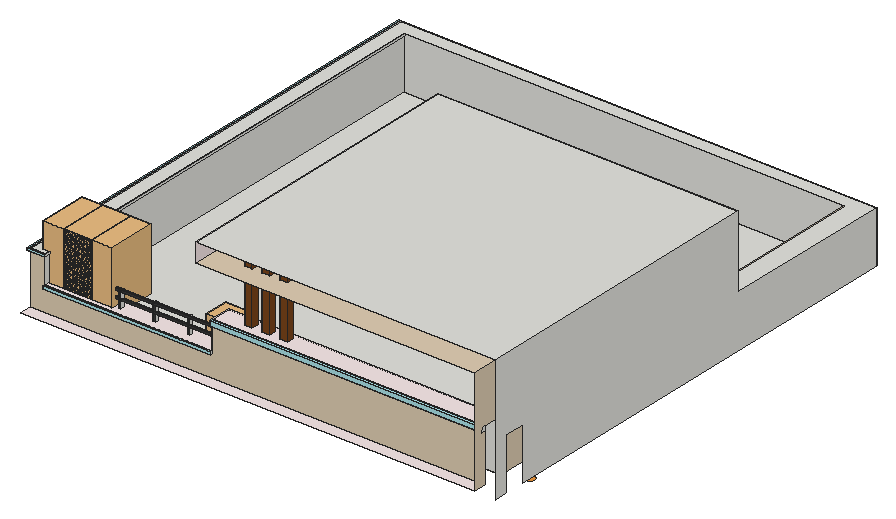
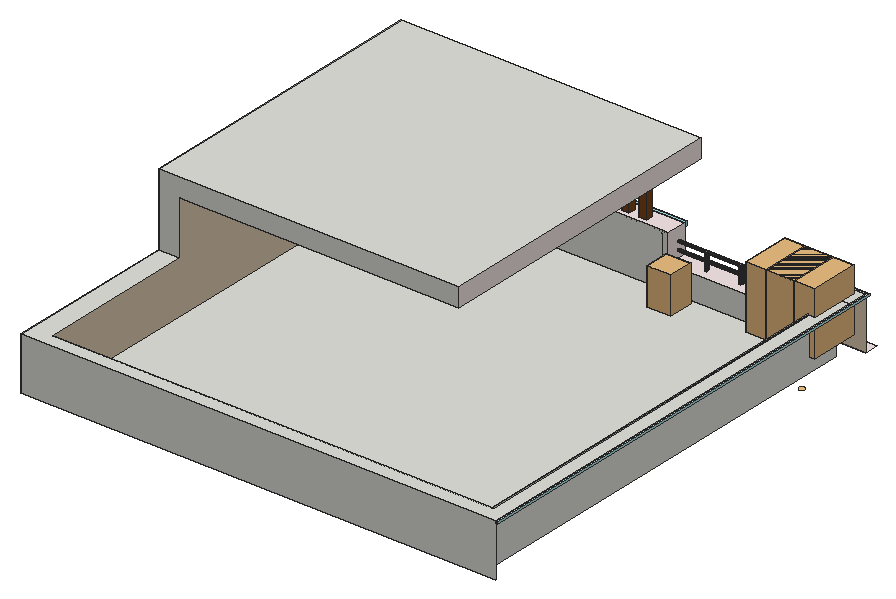
# SketchUp Ruby script. Lengths in inches.
U = 1.inch
M = Sketchup.active_model
def pt(a) = Geom::Point3d.new(a.map { |v| v * U })
def face(e, loops, mat)
  f = e.add_face(loops[0].map { |a| pt(a) })
  loops[1..].each { |l| e.add_face(l.map { |a| pt(a) }).erase! }
  f.material = f.back_material = mat if mat
  f
end
# faces: each face lists its corners as indices into pts; further lists are holes
def faces(e, pts, list, mat = nil) = list.each { |f| face(e, (f[0].is_a?(Array) ? f : [f]).map { |l| l.map { |i| pts[i] } }, mat) }
# xy, xz, yz: faces in a plane at the given z, y or x. An outline is a flat list of corners, or four numbers for a rectangle; further outlines are holes
def ring(l) = l.size == 4 ? [[l[0], l[1]], [l[2], l[1]], [l[2], l[3]], [l[0], l[3]]] : l.each_slice(2).to_a
def flat(e, list, mat, &to3) = list.each { |f| face(e, (f[0].is_a?(Array) ? f : [f]).map { |l| ring(l).map { |u, v| to3.(u, v) } }, mat) }
def xy(e, z, list, mat = nil) = flat(e, list, mat) { |x, y| [x, y, z] }
def xz(e, y, list, mat = nil) = flat(e, list, mat) { |x, z| [x, y, z] }
def yz(e, x, list, mat = nil) = flat(e, list, mat) { |y, z| [x, y, z] }
def lines(e, pts, list) = list.each { |a, b| e.add_line(pt(pts[a]), pt(pts[b])) }
# prism: a flat outline (further loops are holes) pulled along v
def prism(e, loops, v, mat = nil)
  f = face(e, loops, mat); d = Geom::Vector3d.new(v.map { |x| x * U })
  f.pushpull(f.normal.samedirection?(d) ? d.length : -d.length)
end
def box(e, o, s, mat = nil) = prism(e, [[o, [o[0] + s[0], o[1], o[2]], [o[0] + s[0], o[1] + s[1], o[2]], [o[0], o[1] + s[1], o[2]]]], [0, 0, s[2]], mat)
def at(x, y, z, deg = 0) = Geom::Transformation.translation(pt([x, y, z])) * Geom::Transformation.rotation(ORIGIN, Z_AXIS, deg.degrees)
def axes(o, x, y, z) = Geom::Transformation.new([*x, 0, *y, 0, *z, 0, *pt(o).to_a, 1])
def part(name) = M.definitions.add(name)
# library, detail: a bought-in or finely detailed component or shape, given as its bounding box
def library(name, o, s) = part(name).tap { |d| box(d.entities, o, s) }
def detail(e, o, s) = box(e.add_group.entities, o, s)
def put(e, d, t, mat = nil) = e.add_instance(d, t).tap { |i| i.material = mat if mat }
def group(e, t, mat = nil) = e.add_group.tap { |g| g.transformation = t; g.material = mat if mat }.entities
root = M.entities
M.materials.add("Generic\#1").color = [121, 68, 27]
M.materials.add("Generic\#2").color = [245, 199, 133]
M.materials.add("Generic\#4").color = [232, 149, 60]
M.materials.add("Generic\#6").color = [223, 205, 179]
M.materials.add("Generic\#7").color = [171, 227, 232]
M.materials.add("Generic\#9").color = [246, 231, 231]
M.materials.add("[Color M07]").color = [58, 58, 58]
c1 = library("Raised potted plant",[1.65,0,0],[13.63,13.63,20.73])
c2 = library("Plant+2 (1)",[-9.13,-9.52,0],[51.76,51.77,66.88])
c3 = library("Tlon Light 450 Ceiling 152 006",[-8.86,-8.86,-3.78],[17.72,17.72,3.56])
xy(root,545.1875,[[26.07,107.35,25.33,107.49,24.65,107.8,24.07,108.29,23.64,108.9,23.39,109.61,23.32,110.36,23.46,111.1,23.77,111.78,24.26,112.35,24.875,112.78,25.58,113.03,26.33,113.1,27.07,112.97,27.75,112.65,28.32,112.16,28.75,111.55,29,110.84,29.07,110.1,28.9375,109.36,28.62,108.68,28.13,108.1,27.52,107.67,26.8125,107.42],[102.38,107.35,101.64,107.49,100.96,107.8,100.39,108.29,99.96,108.9,99.7,109.61,99.64,110.36,99.77,111.1,100.09,111.78,100.57,112.35,101.1875,112.78,101.89,113.03,102.64,113.1,103.38,112.97,104.06,112.65,104.63,112.16,105.0625,111.55,105.32,110.84,105.38,110.1,105.25,109.36,104.93,108.68,104.45,108.1,103.83,107.67,103.125,107.42],[179.07,107.35,178.33,107.49,177.65,107.8,177.07,108.29,176.64,108.9,176.39,109.61,176.32,110.36,176.46,111.1,176.77,111.78,177.26,112.35,177.875,112.78,178.58,113.03,179.33,113.1,180.07,112.97,180.75,112.65,181.32,112.16,181.75,111.55,182,110.84,182.07,110.1,181.9375,109.36,181.62,108.68,181.13,108.1,180.52,107.67,179.8125,107.42]],"Generic\#2")
xy(root,545.1875,[[327.25,107.79,326.17,108.08,325.19,108.65,324.4,109.45,323.83,110.42,323.54,111.51,323.55,112.64,323.84,113.72,324.4,114.7,325.2,115.49,326.18,116.05,327.26,116.34,328.39,116.34,329.48,116.05,330.45,115.48,331.25,114.6875,331.81,113.71,332.1,112.625,332.1,111.5,331.8,110.41,331.24,109.4375,330.44,108.64,329.47,108.08,328.38,107.79],[417.81,107.79,416.73,108.08,415.75,108.65,414.96,109.45,414.4,110.42,414.11,111.51,414.11,112.64,414.4,113.72,414.97,114.7,415.76,115.49,416.74,116.05,417.83,116.34,418.95,116.34,420.04,116.05,421.01,115.48,421.81,114.6875,422.37,113.71,422.66,112.625,422.66,111.5,422.37,110.41,421.8,109.4375,421,108.64,420.03,108.08,418.94,107.79],[487.25,107.79,486.17,108.08,485.19,108.65,484.4,109.45,483.83,110.42,483.54,111.51,483.55,112.64,483.84,113.72,484.4,114.7,485.2,115.49,486.18,116.05,487.26,116.34,488.39,116.34,489.48,116.05,490.45,115.48,491.25,114.6875,491.81,113.71,492.1,112.625,492.1,111.5,491.8,110.41,491.24,109.4375,490.44,108.64,489.47,108.08,488.38,107.79]],"Generic\#4")
xy(root,563.5,[[17.125,76.4375,485.375,531.65]])
xy(root,563.5,[[2.3125,41,485.375,54.5625]],"Generic\#9")
xy(root,586.375,[[17.125,52.375,195.51,54.5625]])
xy(root,589.5625,[[53.47,63.23,55.65,65.98],[89.68,63.23,91.87,65.98],[125.9,63.23,128.08,65.98],[162.11,63.23,164.3,65.98]])
xy(root,589.5625,[[17.125,52.375,195.51,54.5625]],"Generic\#7")
xy(root,589.5625,[[[17.125,54.5625,195.51,76.4375],[162.11,63.23,164.3,65.98],[125.9,63.23,128.08,65.98],[89.68,63.23,91.87,65.98],[53.47,63.23,55.65,65.98]]],"Generic\#9")
xy(root,607.28,[[53.47,63.23,55.65,65.98],[89.68,63.23,91.87,65.98],[125.9,63.23,128.08,65.98],[162.11,63.23,164.3,65.98]],"[Color M07]")
xy(root,615,[[195.51,50.875,485.375,54.5625]])
xy(root,617.375,[[0,52.5,2.3125,546.8125],[2.3125,52.5,2.3125,54.5625,17.125,54.5625,17.125,531.65,18.6875,531.65,18.6875,52.5]])
xy(root,619.375,[[0,52.5,18.6875,52.5,18.6875,531.65,17.125,531.65,17.125,54.5625,2.3125,54.5625,2.3125,546.8125,0,546.8125],[2.3125,54.5625,17.125,76.4375],[2.3125,76.4375,17.125,76.4375,17.125,531.65,485.375,531.65,485.375,363.375,507.875,363.375,507.875,546.8125,2.3125,546.8125]])
xy(root,619.375,[[195.51,50.875,485.375,54.5625]],"Generic\#7")
xy(root,619.375,[[[195.51,54.5625,485.375,76.4375],[222.76,63.63,230.88,70.88],[241.38,63.63,249.51,70.88],[260.01,63.63,268.13,70.88]]],"Generic\#9")
xy(root,676.25,[[205.79,89.28,204.45,89.45,203.2,89.97,202.125,90.79,201.3,91.87,200.78,93.12,200.6,94.46,200.78,95.81,201.3,97.06,202.125,98.13,203.2,98.96,204.45,99.47,205.79,99.65,207.13,99.47,208.39,98.96,209.46,98.13,210.28,97.06,210.8,95.81,210.98,94.46,210.8,93.12,210.28,91.87,209.46,90.79,208.39,89.97,207.13,89.45]])
xy(root,676.25,[[[188.57,41,485.375,363.375],[291.79,89.28,293.13,89.45,294.39,89.97,295.46,90.79,296.28,91.87,296.8,93.12,296.98,94.46,296.8,95.81,296.28,97.06,295.46,98.13,294.39,98.96,293.13,99.47,291.79,99.65,290.45,99.47,289.2,98.96,288.125,98.13,287.3,97.06,286.78,95.81,286.6,94.46,286.78,93.12,287.3,91.87,288.125,90.79,289.2,89.97,290.45,89.45],[346.04,89.28,347.38,89.45,348.64,89.97,349.71,90.79,350.53,91.87,351.05,93.12,351.23,94.46,351.05,95.81,350.53,97.06,349.71,98.13,348.64,98.96,347.38,99.47,346.04,99.65,344.7,99.47,343.45,98.96,342.375,98.13,341.55,97.06,341.03,95.81,340.85,94.46,341.03,93.12,341.55,91.87,342.375,90.79,343.45,89.97,344.7,89.45],[400.29,89.28,401.63,89.45,402.89,89.97,403.96,90.79,404.78,91.87,405.3,93.12,405.48,94.46,405.3,95.81,404.78,97.06,403.96,98.13,402.89,98.96,401.63,99.47,400.29,99.65,398.95,99.47,397.7,98.96,396.625,98.13,395.8,97.06,395.28,95.81,395.1,94.46,395.28,93.12,395.8,91.87,396.625,90.79,397.7,89.97,398.95,89.45],[454.54,89.28,455.88,89.45,457.14,89.97,458.21,90.79,459.03,91.87,459.55,93.12,459.73,94.46,459.55,95.81,459.03,97.06,458.21,98.13,457.14,98.96,455.88,99.47,454.54,99.65,453.2,99.47,451.95,98.96,450.875,98.13,450.05,97.06,449.53,95.81,449.35,94.46,449.53,93.12,450.05,91.87,450.875,90.79,451.95,89.97,453.2,89.45],[205.79,89.28,207.13,89.45,208.39,89.97,209.46,90.79,210.28,91.87,210.8,93.12,210.98,94.46,210.8,95.81,210.28,97.06,209.46,98.13,208.39,98.96,207.13,99.47,205.79,99.65,204.45,99.47,203.2,98.96,202.125,98.13,201.3,97.06,200.78,95.81,200.6,94.46,200.78,93.12,201.3,91.87,202.125,90.79,203.2,89.97,204.45,89.45]]],"Generic\#6")
xy(root,678.8125,[[291.79,89.28,290.45,89.45,289.2,89.97,288.125,90.79,287.3,91.87,286.78,93.12,286.6,94.46,286.78,95.81,287.3,97.06,288.125,98.13,289.2,98.96,290.45,99.47,291.79,99.65,293.13,99.47,294.39,98.96,295.46,98.13,296.28,97.06,296.8,95.81,296.98,94.46,296.8,93.12,296.28,91.87,295.46,90.79,294.39,89.97,293.13,89.45],[346.04,89.28,344.7,89.45,343.45,89.97,342.375,90.79,341.55,91.87,341.03,93.12,340.85,94.46,341.03,95.81,341.55,97.06,342.375,98.13,343.45,98.96,344.7,99.47,346.04,99.65,347.38,99.47,348.64,98.96,349.71,98.13,350.53,97.06,351.05,95.81,351.23,94.46,351.05,93.12,350.53,91.87,349.71,90.79,348.64,89.97,347.38,89.45],[400.29,89.28,398.95,89.45,397.7,89.97,396.625,90.79,395.8,91.87,395.28,93.12,395.1,94.46,395.28,95.81,395.8,97.06,396.625,98.13,397.7,98.96,398.95,99.47,400.29,99.65,401.63,99.47,402.89,98.96,403.96,98.13,404.78,97.06,405.3,95.81,405.48,94.46,405.3,93.12,404.78,91.87,403.96,90.79,402.89,89.97,401.63,89.45],[454.54,89.28,453.2,89.45,451.95,89.97,450.875,90.79,450.05,91.87,449.53,93.12,449.35,94.46,449.53,95.81,450.05,97.06,450.875,98.13,451.95,98.96,453.2,99.47,454.54,99.65,455.88,99.47,457.14,98.96,458.21,98.13,459.03,97.06,459.55,95.81,459.73,94.46,459.55,93.12,459.03,91.87,458.21,90.79,457.14,89.97,455.88,89.45]],"Generic\#2")
xy(root,682.5,[[222.76,63.63,230.88,70.88],[241.38,63.63,249.51,70.88],[260.01,63.63,268.13,70.88]])
xy(root,696.375,[[188.57,41,507.875,363.375]])
xz(root,50.875,[[195.51,615,485.375,619.375]],"Generic\#7")
xz(root,52.375,[[17.125,586.375,195.51,589.5625]],"Generic\#7")
xz(root,52.5,[[0,617.375,18.6875,619.375]],"Generic\#7")
xz(root,54.5625,[[17.125,586.375,195.51,589.5625],[195.51,615,485.375,619.375],[2.3125,617.375,17.125,619.375]])
xz(root,54.5625,[[2.3125,563.5,485.375,563.5,485.375,615,195.51,615,195.51,586.375,17.125,586.375,17.125,617.375,2.3125,617.375]],"Generic\#6")
xz(root,63.23,[[53.47,589.5625,55.65,607.28],[89.68,589.5625,91.87,607.28],[125.9,589.5625,128.08,607.28],[162.11,589.5625,164.3,607.28]],"[Color M07]")
xz(root,63.63,[[222.76,619.375,230.88,682.5],[241.38,619.375,249.51,682.5],[260.01,619.375,268.13,682.5]],"Generic\#1")
xz(root,65.98,[[53.47,589.5625,55.65,607.28],[89.68,589.5625,91.87,607.28],[125.9,589.5625,128.08,607.28],[162.11,589.5625,164.3,607.28]],"[Color M07]")
xz(root,70.88,[[222.76,619.375,230.88,682.5],[241.38,619.375,249.51,682.5],[260.01,619.375,268.13,682.5]],"Generic\#1")
xz(root,76.4375,[[17.125,563.5,17.125,589.5625,195.51,589.5625,195.51,619.375,201.87,619.375,201.87,563.5],[201.87,563.5,485.375,619.375]])
xz(root,363.375,[[485.375,619.375,485.375,676.25,188.57,676.25,188.57,696.375,507.875,696.375,507.875,619.375]])
xz(root,531.65,[[17.125,563.5,485.375,563.5,485.375,619.375,18.6875,619.375,18.6875,617.375,17.125,617.375]])
xz(root,546.8125,[[2.3125,563.5,507.875,619.375],[0,617.375,2.3125,619.375]])
yz(root,0,[[52.5,617.375,546.8125,619.375]],"Generic\#7")
yz(root,2.3125,[[54.5625,617.375,546.8125,619.375]])
yz(root,17.125,[[76.4375,563.5,531.65,617.375],[[54.5625,589.5625,76.4375,617.375],[62.84,597.4,62.86,599.33,64.97,599.34,64.96,597.42],[62.84,605.34,62.86,607.27,64.97,607.28,64.96,605.36]],[54.5625,617.375,76.4375,619.375],[76.4375,617.375,531.65,619.375]])
yz(root,17.125,[[52.375,586.375,54.5625,589.5625]],"Generic\#7")
yz(root,18.6875,[[52.5,617.375,531.65,619.375]])
yz(root,53.47,[[63.23,589.5625,65.98,607.28]],"[Color M07]")
yz(root,55.65,[[63.23,589.5625,65.98,607.28]])
yz(root,89.68,[[63.23,589.5625,65.98,607.28]],"[Color M07]")
yz(root,91.87,[[63.23,589.5625,65.98,607.28]])
yz(root,125.9,[[63.23,589.5625,65.98,607.28]],"[Color M07]")
yz(root,128.08,[[63.23,589.5625,65.98,607.28]])
yz(root,162.11,[[63.23,589.5625,65.98,607.28]],"[Color M07]")
yz(root,164.3,[[63.23,589.5625,65.98,607.28]])
yz(root,188.57,[[41,676.25,363.375,696.375]],"Generic\#9")
yz(root,195.51,[[52.375,586.375,54.5625,589.5625],[62.84,597.4,64.96,597.42,64.97,599.34,62.86,599.33],[62.84,605.34,64.96,605.36,64.97,607.28,62.86,607.27]])
yz(root,195.51,[[50.875,615,54.5625,619.375]],"Generic\#7")
yz(root,195.51,[[[54.5625,589.5625,76.4375,619.375],[62.84,605.34,64.96,605.36,64.97,607.28,62.86,607.27],[62.84,597.4,64.96,597.42,64.97,599.34,62.86,599.33]]],"Generic\#9")
yz(root,222.76,[[63.63,619.375,70.88,682.5]],"Generic\#1")
yz(root,230.88,[[63.63,619.375,70.88,682.5]],"Generic\#1")
yz(root,241.38,[[63.63,619.375,70.88,682.5]],"Generic\#1")
yz(root,249.51,[[63.63,619.375,70.88,682.5]],"Generic\#1")
yz(root,260.01,[[63.63,619.375,70.88,682.5]],"Generic\#1")
yz(root,268.13,[[63.63,619.375,70.88,682.5]],"Generic\#1")
yz(root,485.375,[[50.875,615,54.5625,619.375]])
yz(root,485.375,[[41,563.5,41,676.25,363.375,676.25,363.375,619.375,531.65,619.375,531.65,563.5,76.4375,563.5,76.4375,619.375,50.875,619.375,50.875,615,54.5625,615,54.5625,563.5]],"Generic\#6")
yz(root,507.875,[[41,563.5,54.5625,563.5,54.5625,619.375,76.4375,619.375,76.4375,563.5,546.8125,563.5,546.8125,619.375,363.375,619.375,363.375,696.375,41,696.375]])
p = [[195.51,62.84,597.4],[195.51,62.86,599.33],[17.125,62.86,599.33],[17.125,62.84,597.4],[195.51,64.96,597.42],[17.125,64.96,597.42],
  [195.51,64.97,599.34],[17.125,64.97,599.34],[195.51,62.84,605.34],[195.51,62.86,607.27],[17.125,62.86,607.27],[17.125,62.84,605.34],
  [195.51,64.96,605.36],[17.125,64.96,605.36],[195.51,64.97,607.28],[17.125,64.97,607.28],[53.47,64.97,607.28],[55.65,64.97,607.28],
  [89.68,64.97,607.28],[91.87,64.97,607.28],[125.9,64.97,607.28],[128.08,64.97,607.28],[162.11,64.97,607.28],[164.3,64.97,607.28],
  [291.79,89.28,676.25],[290.45,89.45,676.25],[290.45,89.45,678.8125],[291.79,89.28,678.8125],[293.13,89.45,676.25],[293.13,89.45,678.8125],
  [346.04,89.28,676.25],[344.7,89.45,676.25],[344.7,89.45,678.8125],[346.04,89.28,678.8125],[347.38,89.45,676.25],[347.38,89.45,678.8125],
  [400.29,89.28,676.25],[398.95,89.45,676.25],[398.95,89.45,678.8125],[400.29,89.28,678.8125],[401.63,89.45,676.25],[401.63,89.45,678.8125],
  [454.54,89.28,676.25],[453.2,89.45,676.25],[453.2,89.45,678.8125],[454.54,89.28,678.8125],[455.88,89.45,676.25],[455.88,89.45,678.8125],
  [289.2,89.97,676.25],[289.2,89.97,678.8125],[294.39,89.97,676.25],[294.39,89.97,678.8125],[343.45,89.97,676.25],[343.45,89.97,678.8125],
  [348.64,89.97,676.25],[348.64,89.97,678.8125],[397.7,89.97,676.25],[397.7,89.97,678.8125],[402.89,89.97,676.25],[402.89,89.97,678.8125],
  [451.95,89.97,676.25],[451.95,89.97,678.8125],[457.14,89.97,676.25],[457.14,89.97,678.8125],[288.125,90.79,676.25],[288.125,90.79,678.8125],
  [295.46,90.79,676.25],[295.46,90.79,678.8125],[342.375,90.79,676.25],[342.375,90.79,678.8125],[349.71,90.79,676.25],[349.71,90.79,678.8125],
  [396.625,90.79,676.25],[396.625,90.79,678.8125],[403.96,90.79,676.25],[403.96,90.79,678.8125],[450.875,90.79,676.25],[450.875,90.79,678.8125],
  [458.21,90.79,676.25],[458.21,90.79,678.8125],[287.3,91.87,676.25],[287.3,91.87,678.8125],[296.28,91.87,676.25],[296.28,91.87,678.8125],
  [341.55,91.87,676.25],[341.55,91.87,678.8125],[350.53,91.87,676.25],[350.53,91.87,678.8125],[395.8,91.87,676.25],[395.8,91.87,678.8125],
  [404.78,91.87,676.25],[404.78,91.87,678.8125],[450.05,91.87,676.25],[450.05,91.87,678.8125],[459.03,91.87,676.25],[459.03,91.87,678.8125],
  [286.78,93.12,676.25],[286.78,93.12,678.8125],[296.8,93.12,676.25],[296.8,93.12,678.8125],[341.03,93.12,676.25],[341.03,93.12,678.8125],
  [351.05,93.12,676.25],[351.05,93.12,678.8125],[395.28,93.12,676.25],[395.28,93.12,678.8125],[405.3,93.12,676.25],[405.3,93.12,678.8125],
  [449.53,93.12,676.25],[449.53,93.12,678.8125],[459.55,93.12,676.25],[459.55,93.12,678.8125],[286.6,94.46,676.25],[286.6,94.46,678.8125],
  [296.98,94.46,676.25],[296.98,94.46,678.8125],[340.85,94.46,676.25],[340.85,94.46,678.8125],[351.23,94.46,676.25],[351.23,94.46,678.8125],
  [395.1,94.46,676.25],[395.1,94.46,678.8125],[405.48,94.46,676.25],[405.48,94.46,678.8125],[449.35,94.46,676.25],[449.35,94.46,678.8125],
  [459.73,94.46,676.25],[459.73,94.46,678.8125],[286.78,95.81,676.25],[286.78,95.81,678.8125],[296.8,95.81,676.25],[296.8,95.81,678.8125],
  [341.03,95.81,676.25],[341.03,95.81,678.8125],[351.05,95.81,676.25],[351.05,95.81,678.8125],[395.28,95.81,676.25],[395.28,95.81,678.8125],
  [405.3,95.81,676.25],[405.3,95.81,678.8125],[449.53,95.81,676.25],[449.53,95.81,678.8125],[459.55,95.81,676.25],[459.55,95.81,678.8125],
  [287.3,97.06,676.25],[287.3,97.06,678.8125],[296.28,97.06,676.25],[296.28,97.06,678.8125],[341.55,97.06,676.25],[341.55,97.06,678.8125],
  [350.53,97.06,676.25],[350.53,97.06,678.8125],[395.8,97.06,676.25],[395.8,97.06,678.8125],[404.78,97.06,676.25],[404.78,97.06,678.8125],
  [450.05,97.06,676.25],[450.05,97.06,678.8125],[459.03,97.06,676.25],[459.03,97.06,678.8125],[288.125,98.13,676.25],[288.125,98.13,678.8125],
  [295.46,98.13,676.25],[295.46,98.13,678.8125],[342.375,98.13,676.25],[342.375,98.13,678.8125],[349.71,98.13,676.25],[349.71,98.13,678.8125],
  [396.625,98.13,676.25],[396.625,98.13,678.8125],[403.96,98.13,676.25],[403.96,98.13,678.8125],[450.875,98.13,676.25],[450.875,98.13,678.8125],
  [458.21,98.13,676.25],[458.21,98.13,678.8125],[289.2,98.96,676.25],[289.2,98.96,678.8125],[294.39,98.96,676.25],[294.39,98.96,678.8125],
  [343.45,98.96,676.25],[343.45,98.96,678.8125],[348.64,98.96,676.25],[348.64,98.96,678.8125],[397.7,98.96,676.25],[397.7,98.96,678.8125],
  [402.89,98.96,676.25],[402.89,98.96,678.8125],[451.95,98.96,676.25],[451.95,98.96,678.8125],[457.14,98.96,676.25],[457.14,98.96,678.8125],
  [290.45,99.47,676.25],[290.45,99.47,678.8125],[293.13,99.47,676.25],[293.13,99.47,678.8125],[344.7,99.47,676.25],[344.7,99.47,678.8125],
  [347.38,99.47,676.25],[347.38,99.47,678.8125],[398.95,99.47,676.25],[398.95,99.47,678.8125],[401.63,99.47,676.25],[401.63,99.47,678.8125],
  [453.2,99.47,676.25],[453.2,99.47,678.8125],[455.88,99.47,676.25],[455.88,99.47,678.8125],[291.79,99.65,676.25],[291.79,99.65,678.8125],
  [346.04,99.65,676.25],[346.04,99.65,678.8125],[400.29,99.65,676.25],[400.29,99.65,678.8125],[454.54,99.65,676.25],[454.54,99.65,678.8125],
  [195.51,63.8,598.36],[17.125,63.8,598.36],[195.51,63.8,606.49],[17.125,63.8,606.49],[163.13,65.01,589.5625],[163.13,65.01,607.28],
  [126.82,65.01,589.5625],[126.82,65.01,607.28],[90.5,65.01,589.5625],[90.5,65.01,607.28],[54.19,65.01,589.5625],[54.19,65.01,607.28]]
faces(root,p,[[0,1,2,3],[6,4,5,7],[1,6,7,2],[8,9,10,11],[14,12,13,15,16,17,18,19,20,21,22,23],[9,14,23,22,21,20,19,18,17,16,15,10]],"[Color M07]")
faces(root,p,[[4,0,3,5],[12,8,11,13]])
faces(root,p,[[24,25,26,27],[28,24,27,29],[30,31,32,33],[34,30,33,35],[36,37,38,39],[40,36,39,41],[42,43,44,45],[46,42,45,47],
  [25,48,49,26],[50,28,29,51],[31,52,53,32],[54,34,35,55],[37,56,57,38],[58,40,41,59],[43,60,61,44],[62,46,47,63],
  [48,64,65,49],[66,50,51,67],[52,68,69,53],[70,54,55,71],[56,72,73,57],[74,58,59,75],[60,76,77,61],[78,62,63,79],
  [64,80,81,65],[82,66,67,83],[68,84,85,69],[86,70,71,87],[72,88,89,73],[90,74,75,91],[76,92,93,77],[94,78,79,95],
  [80,96,97,81],[98,82,83,99],[84,100,101,85],[102,86,87,103],[88,104,105,89],[106,90,91,107],[92,108,109,93],[110,94,95,111],
  [96,112,113,97],[114,98,99,115],[100,116,117,101],[118,102,103,119],[104,120,121,105],[122,106,107,123],[108,124,125,109],[126,110,111,127],
  [112,128,129,113],[130,114,115,131],[116,132,133,117],[134,118,119,135],[120,136,137,121],[138,122,123,139],[124,140,141,125],[142,126,127,143],
  [128,144,145,129],[146,130,131,147],[132,148,149,133],[150,134,135,151],[136,152,153,137],[154,138,139,155],[140,156,157,141],[158,142,143,159],
  [144,160,161,145],[162,146,147,163],[148,164,165,149],[166,150,151,167],[152,168,169,153],[170,154,155,171],[156,172,173,157],[174,158,159,175],
  [160,176,177,161],[178,162,163,179],[164,180,181,165],[182,166,167,183],[168,184,185,169],[186,170,171,187],[172,188,189,173],[190,174,175,191],
  [176,192,193,177],[194,178,179,195],[180,196,197,181],[198,182,183,199],[184,200,201,185],[202,186,187,203],[188,204,205,189],[206,190,191,207],
  [192,208,209,193],[208,194,195,209],[196,210,211,197],[210,198,199,211],[200,212,213,201],[212,202,203,213],[204,214,215,205],[214,206,207,215]],"Generic\#2")
lines(root,p,[[216,217],[218,219],[220,221],[222,223],[224,225],[226,227]])
put(root,c1,axes([164.16,81.93,563.5],[1.8886,0,0],[0,1.8886,0],[0,0,1.8886]))
put(root,c2,at(20.18,69.54,579.29))
put(root,c2,at(42.18,69.54,579.29))
put(root,c3,axes([400.08,94.94,676.24],[0.6431,0,0],[0,0.6431,0],[0,0,0.6431]))
put(root,c3,axes([454.39,94.94,676.24],[0.6431,0,0],[0,0.6431,0],[0,0,0.6431]))
put(root,c3,axes([346.51,94.94,676.24],[0.6431,0,0],[0,0.6431,0],[0,0,0.6431]))
put(root,c3,axes([291.45,94.94,676.24],[0.6431,0,0],[0,0.6431,0],[0,0,0.6431]))
put(root,c3,axes([205.7,94.94,676.24],[0.6431,0,0],[0,0.6431,0],[0,0,0.6431]))
